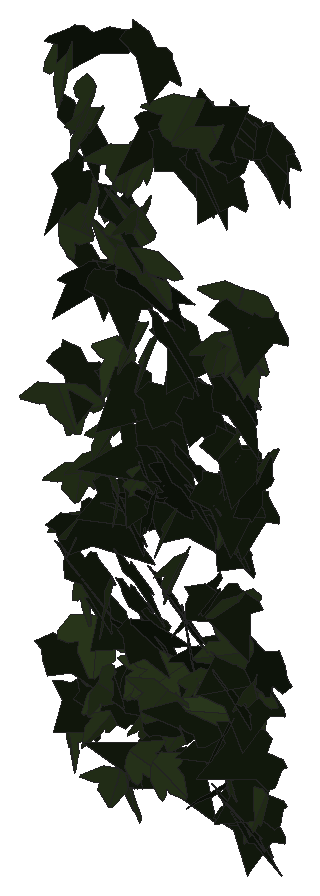
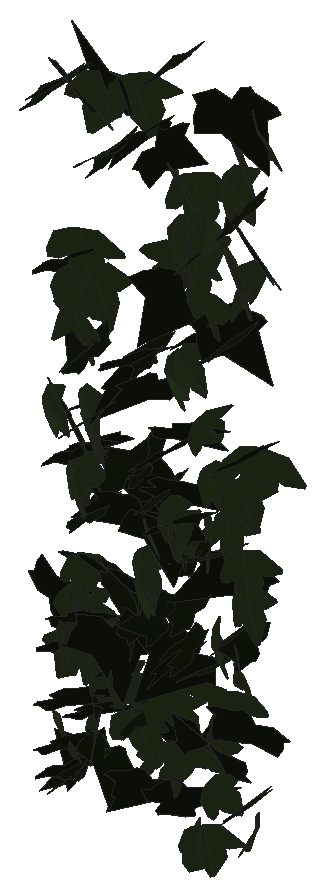
# SketchUp Ruby script. Lengths in inches.
U = 1.inch
M = Sketchup.active_model
def pt(a) = Geom::Point3d.new(a.map { |v| v * U })
def face(e, loops, mat)
  f = e.add_face(loops[0].map { |a| pt(a) })
  loops[1..].each { |l| e.add_face(l.map { |a| pt(a) }).erase! }
  f.material = f.back_material = mat if mat
  f
end
# faces: each face lists its corners as indices into pts; further lists are holes
def faces(e, pts, list, mat = nil) = list.each { |f| face(e, (f[0].is_a?(Array) ? f : [f]).map { |l| l.map { |i| pts[i] } }, mat) }
# xy, xz, yz: faces in a plane at the given z, y or x. An outline is a flat list of corners, or four numbers for a rectangle; further outlines are holes
def ring(l) = l.size == 4 ? [[l[0], l[1]], [l[2], l[1]], [l[2], l[3]], [l[0], l[3]]] : l.each_slice(2).to_a
def flat(e, list, mat, &to3) = list.each { |f| face(e, (f[0].is_a?(Array) ? f : [f]).map { |l| ring(l).map { |u, v| to3.(u, v) } }, mat) }
def xy(e, z, list, mat = nil) = flat(e, list, mat) { |x, y| [x, y, z] }
def xz(e, y, list, mat = nil) = flat(e, list, mat) { |x, z| [x, y, z] }
def yz(e, x, list, mat = nil) = flat(e, list, mat) { |y, z| [x, y, z] }
def lines(e, pts, list) = list.each { |a, b| e.add_line(pt(pts[a]), pt(pts[b])) }
# prism: a flat outline (further loops are holes) pulled along v
def prism(e, loops, v, mat = nil)
  f = face(e, loops, mat); d = Geom::Vector3d.new(v.map { |x| x * U })
  f.pushpull(f.normal.samedirection?(d) ? d.length : -d.length)
end
def box(e, o, s, mat = nil) = prism(e, [[o, [o[0] + s[0], o[1], o[2]], [o[0] + s[0], o[1] + s[1], o[2]], [o[0], o[1] + s[1], o[2]]]], [0, 0, s[2]], mat)
def at(x, y, z, deg = 0) = Geom::Transformation.translation(pt([x, y, z])) * Geom::Transformation.rotation(ORIGIN, Z_AXIS, deg.degrees)
def axes(o, x, y, z) = Geom::Transformation.new([*x, 0, *y, 0, *z, 0, *pt(o).to_a, 1])
def part(name) = M.definitions.add(name)
# library, detail: a bought-in or finely detailed component or shape, given as its bounding box
def library(name, o, s) = part(name).tap { |d| box(d.entities, o, s) }
def detail(e, o, s) = box(e.add_group.entities, o, s)
def put(e, d, t, mat = nil) = e.add_instance(d, t).tap { |i| i.material = mat if mat }
def group(e, t, mat = nil) = e.add_group.tap { |g| g.transformation = t; g.material = mat if mat }.entities
root = M.entities
M.materials.add("1026 AP 7946 SUNNY SIDE UP").color = [254, 231, 186]
M.materials.add("efeu1").color = [18, 25, 13]
M.materials.add("efeu2").color = [43, 57, 29]
c1 = part("ivyleaf_10")
p = [[0,0.5,-0.03],[-0.0625,2.02,-0.43],[-0.19,2.01,-0.46],[-0.54,1.05,-0.29],[-0.52,0.625,-0.18],[-0.83,0.76,-0.28],
  [-1.16,0.64,-0.33],[-1.15,0.33,-0.24],[-0.77,-0.39,0.02],[-0.3,-0.51,0.16],[0.04,-0.48,0.23],[-0.02,2.01,-0.4375],
  [-0.06,2.01,-0.43],[0.04,-0.49,0.23],[0.67,-0.49,0.14],[1.38,0.36,-0.2],[1.375,0.51,-0.24],[0.81,0.65,-0.19],
  [0.62,0.59,-0.15],[0.6,1.09,-0.28],[0.5,1.23,-0.31]]
faces(c1.entities,p,[[0,1,2,3,4,5,6,7,8,9,10],[11,12,0,13,14,15,16,17,18,19,20]],"efeu2")
c2 = part("ivyleaf_9")
p = [[1.54,2.16,1.25],[1.36,2.04,1.19],[-0.21,0.99,0.68],[-0.71,1.11,0.82],[-0.85,0.86,0.67],[-0.8,0.17,0.21],
  [-0.9,-0.01,0.1],[-0.67,-0.16,-0.02],[-0.08,-0.08,-0.05],[-0.03,-0.6,-0.4],[0.65,-0.88,-0.66],[0.83,-0.6,-0.49],
  [1.29,-0.42,-0.43],[1.8125,-0.07,-0.26],[1.21,0.44,0.15]]
faces(c2.entities,p,[[0,1,2,3,4,5,6,7,8,9,10,11,12,13,14]],"efeu1")
put(root,c1,axes([114.49,211.98,276.21],[-0.46755,0.04693,-0.12502],[0.17989,-0.05127,-0.30883],[-0.09827,-0.31714,0.02948]),"1026 AP 7946 SUNNY SIDE UP")
put(root,c1,axes([113.89,211.85,269.51],[0.00016,-0.20597,-0.21313],[0.10425,0.20032,-0.20542],[0.4457,-0.04678,0.04812]),"1026 AP 7946 SUNNY SIDE UP")
put(root,c1,axes([115.85,212.03,275.45],[-0.07822,-0.31944,0.02119],[0.00362,-0.02301,-0.33313],[0.50351,-0.04946,0.00569]),"1026 AP 7946 SUNNY SIDE UP")
put(root,c2,axes([115.95,212.16,268.2],[0.06977,-0.19538,0.20513],[0.16188,-0.1771,-0.20257],[0.40903,0.10342,0.04518]),"1026 AP 7946 SUNNY SIDE UP")
put(root,c1,axes([114.95,211.84,268.58],[-0.00441,0.23066,0.16475],[-0.00701,0.15856,-0.2367],[-0.44011,-0.00484,0.00212]),"1026 AP 7946 SUNNY SIDE UP")
put(root,c1,axes([113.74,212.17,270.73],[0.17168,-0.16437,0.23033],[0.20283,-0.1838,-0.20433],[0.38768,0.16896,0.0049]),"1026 AP 7946 SUNNY SIDE UP")
put(root,c1,axes([116.42,212.08,268.5],[0.29242,-0.22063,0.0544],[0.03417,-0.05227,-0.29707],[0.35554,0.18648,-0.0162]),"1026 AP 7946 SUNNY SIDE UP")
put(root,c1,axes([114.85,212.02,269.61],[-0.38768,-0.02334,0.12794],[-0.18581,-0.05466,-0.25232],[0.07095,-0.27066,0.03826]),"1026 AP 7946 SUNNY SIDE UP")
put(root,c1,axes([114.54,211.85,268.63],[0.06931,0.17777,0.19827],[-0.0026,0.19434,-0.18437],[-0.41079,0.02876,0.03462]),"1026 AP 7946 SUNNY SIDE UP")
put(root,c2,axes([115.3,211.91,270.875],[0.19725,-0.09015,-0.26132],[-0.36298,0.10687,-0.15643],[0.21631,0.26154,-0.02419]),"1026 AP 7946 SUNNY SIDE UP")
put(root,c2,axes([115.85,212.2,270],[0.04597,-0.18928,0.19439],[0.10568,-0.17961,-0.19628],[0.40798,0.06785,0.02894]),"1026 AP 7946 SUNNY SIDE UP")
put(root,c1,axes([113.11,212,273.67],[-0.42995,-0.14829,-0.06151],[0.10163,0.00382,-0.31922],[0.22936,-0.27967,0.02616]),"1026 AP 7946 SUNNY SIDE UP")
put(root,c2,axes([115.88,212.16,273.05],[-0.12212,-0.27707,-0.02042],[0.01419,0.01643,-0.29631],[0.43638,-0.07807,0.00392]),"1026 AP 7946 SUNNY SIDE UP")
put(root,c2,axes([113.99,212.26,270.3],[-0.22655,-0.15842,0.19485],[-0.02833,-0.21261,-0.19791],[0.38799,-0.10803,0.09932]),"1026 AP 7946 SUNNY SIDE UP")
put(root,c2,axes([114.92,212.12,273.1],[0.24743,-0.23517,0.04497],[0.02039,-0.04538,-0.2914],[0.37593,0.15724,-0.0138]),"1026 AP 7946 SUNNY SIDE UP")
put(root,c1,axes([113.35,212.09,271.72],[0.04268,-0.27673,0.03072],[0.00247,-0.03138,-0.28663],[0.43791,0.02715,-0.00138]),"1026 AP 7946 SUNNY SIDE UP")
put(root,c1,axes([113.49,212.07,278.35],[0.26298,-0.28923,-0.02446],[-0.02518,0.01627,-0.34405],[0.45542,0.16791,-0.0049]),"1026 AP 7946 SUNNY SIDE UP")
put(root,c1,axes([112.97,212.1875,278.73],[0.31753,-0.17989,0.18977],[0.19823,-0.13653,-0.27898],[0.35433,0.23759,-0.01398]),"1026 AP 7946 SUNNY SIDE UP")
put(root,c2,axes([113.3,212.15,277.02],[-0.39035,0.08105,-0.18814],[0.25758,-0.08546,-0.26831],[-0.18102,-0.29639,0.02391]),"1026 AP 7946 SUNNY SIDE UP")
put(root,c2,axes([115.99,211.85,269.45],[-0.12678,0.04384,-0.28372],[-0.32819,0.18103,0.09362],[0.2914,0.22297,-0.01801]),"1026 AP 7946 SUNNY SIDE UP")
put(root,c2,axes([115.53,212.22,269.4],[-0.24623,-0.01333,0.22768],[-0.29463,-0.13639,-0.146],[0.18569,-0.23409,0.07026]),"1026 AP 7946 SUNNY SIDE UP")
put(root,c2,axes([115.97,212.26,273.65],[-0.12615,-0.26399,0.08757],[0.01946,-0.09334,-0.28219],[0.43638,-0.07215,0.0379]),"1026 AP 7946 SUNNY SIDE UP")
put(root,c2,axes([113.375,212.18,271.08],[0.11517,-0.29673,0.00737],[-0.00621,-0.01008,-0.31486],[0.46674,0.07308,-0.00601]),"1026 AP 7946 SUNNY SIDE UP")
put(root,c2,axes([113.64,212.13,275.66],[-0.03296,0.21047,-0.24576],[0.02622,-0.23922,-0.21924],[-0.50095,-0.02637,0.00469]),"1026 AP 7946 SUNNY SIDE UP")
put(root,c2,axes([115.52,212.13,278.375],[-0.12133,0.15289,0.29056],[0.18785,-0.25457,0.17488],[0.46688,0.14216,0.00514]),"1026 AP 7946 SUNNY SIDE UP")
put(root,c2,axes([116.31,212.31,269.12],[-0.31889,-0.14425,0.1828],[-0.18201,-0.14103,-0.25406],[0.31126,-0.23025,0.03871]),"1026 AP 7946 SUNNY SIDE UP")
put(root,c2,axes([114.45,212.3125,279.27],[-0.05763,-0.26594,0.15487],[0.00393,-0.15318,-0.27666],[0.48152,-0.03058,0.02079]),"1026 AP 7946 SUNNY SIDE UP")
put(root,c2,axes([114.01,212.28,272.02],[0.07618,-0.18441,0.21341],[0.06247,-0.20458,-0.1974],[0.43285,0.06198,-0.00907]),"1026 AP 7946 SUNNY SIDE UP")
put(root,c1,axes([115.68,212.07,278.49],[-0.40505,-0.19865,-0.0706],[0.10673,0.02207,-0.33411],[0.3121,-0.26535,0.02263]),"1026 AP 7946 SUNNY SIDE UP")
put(root,c2,axes([114.96,212.25,270.76],[0.30141,-0.09309,-0.20331],[0.29183,-0.06726,0.21858],[-0.17901,-0.26638,0.01401]),"1026 AP 7946 SUNNY SIDE UP")
put(root,c2,axes([116.08,212.11,268.14],[0.28891,-0.18786,-0.04595],[-0.05544,0.02639,-0.27047],[0.29811,0.18697,-0.00577]),"1026 AP 7946 SUNNY SIDE UP")
put(root,c2,axes([113.51,211.96,271.91],[-0.01021,-0.06465,-0.32276],[0.12518,0.3028,-0.06438],[0.48661,-0.07926,0.00979]),"1026 AP 7946 SUNNY SIDE UP")
put(root,c1,axes([115.12,212.18,278.69],[-0.29611,-0.25142,0.09091],[-0.0419,-0.09149,-0.32244],[0.41763,-0.18745,0.0321]),"1026 AP 7946 SUNNY SIDE UP")
put(root,c1,axes([113.31,211.89,276.34],[-0.01347,0.18595,0.27429],[-0.11269,0.25763,-0.18698],[-0.49667,-0.0635,0.03499]),"1026 AP 7946 SUNNY SIDE UP")
put(root,c1,axes([114,212.03,272.41],[0.18204,-0.21785,-0.14607],[-0.00546,0.15261,-0.24574],[0.40762,0.09934,0.06194]),"1026 AP 7946 SUNNY SIDE UP")
put(root,c1,axes([114.22,212.25,274.88],[0.05092,-0.26007,0.14748],[0.04114,-0.14244,-0.27072],[0.46611,0.04098,0.00778]),"1026 AP 7946 SUNNY SIDE UP")
put(root,c1,axes([115.56,212.25,269.5],[-0.08745,0.07249,0.26375],[-0.25602,-0.21566,0.02525],[0.33013,-0.14805,0.08945]),"1026 AP 7946 SUNNY SIDE UP")
put(root,c2,axes([113.88,212.28,275.52],[-0.02287,-0.30449,0.02906],[-0.00042,-0.02996,-0.31422],[0.48109,-0.0145,0.0011]),"1026 AP 7946 SUNNY SIDE UP")
put(root,c1,axes([116.18,212.25,275.45],[-0.10318,-0.24931,0.14987],[-0.03804,-0.14537,-0.26616],[0.45341,-0.06893,0.01178]),"1026 AP 7946 SUNNY SIDE UP")
put(root,c2,axes([116.2,212.27,268.13],[-0.13827,-0.25698,0.015],[0.00443,-0.01789,-0.27978],[0.40484,-0.08758,0.00819]),"1026 AP 7946 SUNNY SIDE UP")
put(root,c2,axes([114.68,212.18,272.68],[0.14344,-0.05207,0.27289],[0.3296,-0.16303,-0.10822],[0.26823,0.22818,-0.01296]),"1026 AP 7946 SUNNY SIDE UP")
put(root,c2,axes([113.07,212.22,271.02],[0.25099,-0.21041,0.08354],[0.05945,-0.07446,-0.27212],[0.35024,0.16342,-0.01368]),"1026 AP 7946 SUNNY SIDE UP")
put(root,c2,axes([115.86,212.34,269.1],[-0.28199,-0.09829,0.18486],[-0.18036,-0.15014,-0.20307],[0.26732,-0.20499,0.05799]),"1026 AP 7946 SUNNY SIDE UP")
put(root,c2,axes([116.32,212.35,268.45],[-0.25498,-0.15213,0.15768],[-0.12726,-0.13574,-0.22686],[0.31559,-0.17765,0.03591]),"1026 AP 7946 SUNNY SIDE UP")
put(root,c1,axes([115.88,212.07,268.78],[-0.2182,0.22179,0.07135],[-0.098,0.04068,-0.26748],[-0.35135,-0.14908,0.03029]),"1026 AP 7946 SUNNY SIDE UP")
put(root,c2,axes([116.17,212.32,275.8],[-0.16645,-0.27761,0.02002],[0.00377,-0.02339,-0.30602],[0.43775,-0.10536,0.01025]),"1026 AP 7946 SUNNY SIDE UP")
put(root,c2,axes([113.15,212.16,269.76],[-0.07612,-0.14172,-0.26228],[0.3244,0.1645,-0.13421],[0.32198,-0.19924,0.07321]),"1026 AP 7946 SUNNY SIDE UP")
put(root,c1,axes([116.09,212.21,270.64],[-0.22466,-0.04339,0.26123],[-0.35516,-0.11827,-0.1525],[0.19443,-0.26617,0.02327]),"1026 AP 7946 SUNNY SIDE UP")
put(root,c2,axes([114.0625,212.28,271.1875],[0.17915,-0.22704,0.11541],[0.06852,-0.10486,-0.2622],[0.39306,0.12176,-0.00689]),"1026 AP 7946 SUNNY SIDE UP")
put(root,c2,axes([113.875,212.29,276.73],[0.10515,-0.29695,0.03704],[-0.00037,-0.03862,-0.31367],[0.47066,0.06631,-0.00852]),"1026 AP 7946 SUNNY SIDE UP")
put(root,c1,axes([115.85,212.32,272.73],[-0.02744,-0.21768,0.19612],[0.0818,-0.19119,-0.22],[0.44859,0.02155,0.05212]),"1026 AP 7946 SUNNY SIDE UP")
put(root,c2,axes([114.39,212.14,269.125],[-0.1717,0.14195,0.27367],[0.29961,-0.18517,0.1821],[0.36534,0.21857,-0.02073]),"1026 AP 7946 SUNNY SIDE UP")
put(root,c2,axes([115.36,212.05,274.29],[0.16756,-0.17896,-0.25689],[-0.19975,0.21339,-0.21332],[0.43791,0.16581,0.00099]),"1026 AP 7946 SUNNY SIDE UP")
put(root,c2,axes([114.95,212.21,278.08],[0.09111,-0.30461,-0.11204],[-0.02654,0.10573,-0.3188],[0.50697,0.06028,0.00345]),"1026 AP 7946 SUNNY SIDE UP")
put(root,c1,axes([114.76,212.28,272.22],[0.16562,-0.23316,0.1238],[0.05849,-0.11636,-0.26393],[0.40925,0.11099,-0.01238]),"1026 AP 7946 SUNNY SIDE UP")
put(root,c1,axes([114.32,212.1,276.54],[-0.29457,0.04892,-0.26597],[-0.36974,0.11106,0.19789],[0.18537,0.29926,-0.02793]),"1026 AP 7946 SUNNY SIDE UP")
put(root,c2,axes([114.85,212.08,274.3],[0.09193,-0.18633,-0.23931],[0.02197,0.23714,-0.19183],[0.46644,0.02556,0.0562]),"1026 AP 7946 SUNNY SIDE UP")
put(root,c1,axes([114.29,212.17,276.77],[-0.00488,-0.31759,-0.0343],[0.00653,0.03145,-0.32699],[0.50179,-0.0035,0.00392]),"1026 AP 7946 SUNNY SIDE UP")
put(root,c1,axes([113.38,212.29,277.87],[0.01818,-0.29185,0.13558],[0.02889,-0.13253,-0.30143],[0.50366,0.01814,0.0124]),"1026 AP 7946 SUNNY SIDE UP")
put(root,c2,axes([116.53,211.97,273.37],[-0.23333,0.04716,-0.30152],[-0.41909,0.12277,0.16017],[0.20506,0.30458,-0.01576]),"1026 AP 7946 SUNNY SIDE UP")
put(root,c2,axes([114.92,212.38,269.25],[-0.05002,-0.17703,0.21674],[0.06438,-0.21347,-0.17907],[0.42876,0.0114,0.05217]),"1026 AP 7946 SUNNY SIDE UP")
put(root,c2,axes([115.62,212.25,271.3125],[-0.1614,-0.17412,-0.20265],[0.31254,0.08516,-0.18493],[0.2683,-0.20394,0.09352]),"1026 AP 7946 SUNNY SIDE UP")
put(root,c2,axes([116.62,212.06,270.43],[0.0342,-0.03002,0.30632],[-0.23398,0.25766,0.0395],[-0.40784,-0.15034,0.00303]),"1026 AP 7946 SUNNY SIDE UP")
put(root,c1,axes([113.77,212.25,273.3],[-0.02669,-0.27337,0.07978],[-0.0086,-0.07881,-0.28263],[0.44736,-0.01782,-0.00067]),"1026 AP 7946 SUNNY SIDE UP")
put(root,c2,axes([116.01,212.33,272.97],[-0.12563,-0.28007,0.01122],[0.00575,-0.01402,-0.30002],[0.44078,-0.07964,0.00711]),"1026 AP 7946 SUNNY SIDE UP")
put(root,c1,axes([114.35,212.34,274.67],[0.18237,-0.206,0.19581],[0.12986,-0.17278,-0.24434],[0.42247,0.14203,-0.00942]),"1026 AP 7946 SUNNY SIDE UP")
put(root,c2,axes([115.83,212.26,274.54],[0.11102,-0.27987,-0.03842],[-0.03125,0.03178,-0.29694],[0.44253,0.07246,-0.01133]),"1026 AP 7946 SUNNY SIDE UP")
put(root,c2,axes([114.41,212.08,275.81],[0.46875,0.06205,-0.05582],[-0.07525,-0.03675,-0.31278],[-0.10587,0.30082,-0.02484]),"1026 AP 7946 SUNNY SIDE UP")
put(root,c1,axes([114.92,212.23,271.625],[0.01355,-0.29129,0.02442],[-0.00187,-0.02541,-0.30036],[0.45975,0.00848,-0.00194]),"1026 AP 7946 SUNNY SIDE UP")
put(root,c2,axes([116.05,212.36,270.45],[-0.34372,-0.15109,0.09497],[-0.09282,-0.07731,-0.27264],[0.26312,-0.22464,0.02788]),"1026 AP 7946 SUNNY SIDE UP")
put(root,c2,axes([116.06,212.31,269.99],[-0.23945,-0.22061,-0.06469],[0.09933,0.03058,-0.27378],[0.34616,-0.16138,0.03381]),"1026 AP 7946 SUNNY SIDE UP")
put(root,c1,axes([113.51,212.22,270.08],[0.47409,0.09148,0.01457],[0.03107,-0.01834,-0.32381],[-0.14206,0.30126,-0.02221]),"1026 AP 7946 SUNNY SIDE UP")
put(root,c2,axes([115.68,212.02,268.43],[0.04162,0.26217,0.06305],[0.00271,0.05984,-0.27107],[-0.42279,0.02619,0.00447]),"1026 AP 7946 SUNNY SIDE UP")
put(root,c1,axes([116.02,212.21,276.08],[-0.41937,-0.11855,0.05922],[-0.06287,-0.05242,-0.29928],[0.19788,-0.26789,0.03043]),"1026 AP 7946 SUNNY SIDE UP")
put(root,c1,axes([114.35,212.26,277.66],[0.33162,-0.27042,0.01062],[-0.01148,-0.0207,-0.3529],[0.42546,0.21021,-0.0178]),"1026 AP 7946 SUNNY SIDE UP")
put(root,c1,axes([114.06,212.22,277.59],[-0.28765,-0.2639,0.01735],[0.01065,-0.02697,-0.33026],[0.41582,-0.18187,0.02047]),"1026 AP 7946 SUNNY SIDE UP")
put(root,c1,axes([114.8,212.25,269.87],[0.40913,-0.00443,-0.15975],[-0.24331,-0.02812,-0.26687],[-0.01668,0.30158,-0.02546]),"1026 AP 7946 SUNNY SIDE UP")
put(root,c2,axes([114.26,212.09,270.41],[0.48433,0.08456,-0.00381],[0.00611,-0.02987,-0.3278],[-0.13298,0.3066,-0.02894]),"1026 AP 7946 SUNNY SIDE UP")
put(root,c2,axes([115.72,212.4375,272.09],[-0.13274,-0.1676,0.22981],[0.011,-0.2352,-0.17993],[0.43979,-0.04471,0.07386]),"1026 AP 7946 SUNNY SIDE UP")
put(root,c1,axes([115.07,212.23,269.18],[-0.33823,-0.121,0.10108],[-0.12385,-0.0612,-0.25422],[0.21213,-0.22866,0.01274]),"1026 AP 7946 SUNNY SIDE UP")
put(root,c2,axes([113.98,212.42,272.08],[-0.32255,-0.09937,0.16937],[-0.08355,-0.20247,-0.19488],[0.29107,-0.16823,0.13175]),"1026 AP 7946 SUNNY SIDE UP")
put(root,c2,axes([115.51,212.4375,277.66],[-0.16719,-0.24119,0.15279],[-0.02479,-0.15457,-0.26904],[0.44566,-0.09908,0.04235]),"1026 AP 7946 SUNNY SIDE UP")
put(root,c2,axes([114.53,212.43,278.1],[-0.00969,0.00304,-0.334],[0.19043,-0.3008,-0.00703],[-0.47294,-0.12118,0.00401]),"1026 AP 7946 SUNNY SIDE UP")
put(root,c1,axes([113.17,212.25,271.66],[-0.06525,-0.28072,0.02025],[0.0005,-0.02152,-0.29244],[0.44266,-0.04135,0.00332]),"1026 AP 7946 SUNNY SIDE UP")
put(root,c2,axes([114.26,212.4,273.94],[-0.36925,-0.15721,0.06137],[-0.05208,-0.05861,-0.28987],[0.25968,-0.2353,0.02913]),"1026 AP 7946 SUNNY SIDE UP")
put(root,c2,axes([114.33,212.18,270.41],[0.13926,-0.21898,-0.19317],[-0.09873,0.17546,-0.24224],[0.44113,0.1084,0.00676]),"1026 AP 7946 SUNNY SIDE UP")
put(root,c1,axes([115.82,212.28,273.42],[0.17046,-0.26571,0.0245],[0.00222,-0.02673,-0.29566],[0.41969,0.10806,-0.00839]),"1026 AP 7946 SUNNY SIDE UP")
put(root,c1,axes([113.49,212.22,272.73],[-0.11207,-0.27856,-0.04915],[0.03912,0.04119,-0.29564],[0.44225,-0.07423,0.01369]),"1026 AP 7946 SUNNY SIDE UP")
put(root,c1,axes([116.25,212.16,270.2],[-0.02326,-0.24599,-0.14891],[0.02981,0.14217,-0.25287],[0.44652,-0.0223,0.00912]),"1026 AP 7946 SUNNY SIDE UP")
put(root,c2,axes([114.46,212.37,268.23],[-0.11768,0.0014,0.27317],[-0.3952,-0.08818,-0.07312],[0.13287,-0.26103,0.02446]),"1026 AP 7946 SUNNY SIDE UP")
put(root,c1,axes([115.22,212.375,269.85],[-0.01196,-0.2398,0.14704],[0.02597,-0.14428,-0.2473],[0.43913,0.00201,0.01863]),"1026 AP 7946 SUNNY SIDE UP")
put(root,c1,axes([114.45,212.36,269.7],[-0.27173,-0.11601,0.1695],[-0.12579,-0.16029,-0.20312],[0.29141,-0.17737,0.07037]),"1026 AP 7946 SUNNY SIDE UP")
put(root,c1,axes([116.05,212.26,272.58],[0.04387,-0.2895,-0.02645],[-0.0055,0.02381,-0.29948],[0.45674,0.02809,-0.00107]),"1026 AP 7946 SUNNY SIDE UP")
put(root,c2,axes([115.43,212.33,271.28],[-0.29415,0.14107,-0.15837],[0.16168,-0.11855,-0.24042],[-0.28654,-0.21171,0.02692]),"1026 AP 7946 SUNNY SIDE UP")
put(root,c1,axes([116.07,212.25,274.94],[0.3506,-0.17854,-0.08279],[-0.08158,0.06198,-0.29348],[0.29618,0.22841,0.01717]),"1026 AP 7946 SUNNY SIDE UP")
put(root,c2,axes([115.75,212.48,273.56],[-0.09297,-0.25627,0.14066],[-0.0266,-0.13754,-0.27143],[0.4569,-0.06015,0.01282]),"1026 AP 7946 SUNNY SIDE UP")
put(root,c1,axes([113.17,212.38,270.64],[0.21838,-0.13518,0.20239],[0.25222,-0.11647,-0.19929],[0.27882,0.21124,0.02176]),"1026 AP 7946 SUNNY SIDE UP")
put(root,c1,axes([113.4,212.27,276.66],[0.2788,-0.27954,-0.07121],[-0.06076,0.05547,-0.34069],[0.4481,0.18145,-0.00189]),"1026 AP 7946 SUNNY SIDE UP")
put(root,c1,axes([113.58,212.42,268.72],[-0.05823,-0.18897,0.19337],[0.00171,-0.19069,-0.19755],[0.42,-0.02542,0.02761]),"1026 AP 7946 SUNNY SIDE UP")
put(root,c2,axes([114.49,212.4,272.96],[-0.40496,-0.03107,0.1612],[-0.23685,-0.05152,-0.26594],[0.08345,-0.29701,0.02746]),"1026 AP 7946 SUNNY SIDE UP")
put(root,c2,axes([113.15,212.46,273.9],[-0.10284,-0.27208,0.0823],[-0.00553,-0.08279,-0.28833],[0.44654,-0.06369,0.01539]),"1026 AP 7946 SUNNY SIDE UP")
put(root,c1,axes([113.83,212.3,267.91],[-0.28729,-0.18059,0.03552],[-0.02196,-0.03628,-0.26436],[0.28856,-0.18255,0.01525]),"1026 AP 7946 SUNNY SIDE UP")
put(root,c2,axes([115.03,212.46,273.01],[0.063,-0.22576,0.19194],[0.12793,-0.17337,-0.23386],[0.44346,0.08208,0.0402]),"1026 AP 7946 SUNNY SIDE UP")
put(root,c1,axes([113.71,212.37,269.25],[0.25873,0.13618,-0.1651],[-0.1825,-0.11206,-0.22046],[-0.27688,0.20112,-0.00897]),"1026 AP 7946 SUNNY SIDE UP")
put(root,c1,axes([114.3125,212.4375,272.66],[-0.02573,-0.21482,0.18919],[0.02007,-0.18554,-0.22204],[0.44519,-0.00405,0.02094]),"1026 AP 7946 SUNNY SIDE UP")
put(root,c2,axes([113.11,212.51,268.6],[-0.16046,-0.14633,0.21381],[-0.06959,-0.21088,-0.17612],[0.39428,-0.09677,0.05593]),"1026 AP 7946 SUNNY SIDE UP")
put(root,c1,axes([112.98,212.34,268.3125],[-0.06259,0.23569,-0.11815],[0.03526,-0.11387,-0.24689],[-0.41157,-0.0456,-0.00318]),"1026 AP 7946 SUNNY SIDE UP")
put(root,c2,axes([115.875,212.3,268.26],[0.16988,-0.21924,-0.08883],[-0.04311,0.08114,-0.25108],[0.3672,0.11095,0.01162]),"1026 AP 7946 SUNNY SIDE UP")
put(root,c2,axes([114.59,212.42,274.98],[0.17144,-0.26375,0.07378],[0.02641,-0.0721,-0.29419],[0.42954,0.1097,-0.01136]),"1026 AP 7946 SUNNY SIDE UP")
put(root,c2,axes([115.26,212.46,277.76],[0.08598,-0.28808,0.07874],[0.008,-0.07845,-0.30238],[0.46925,0.05412,-0.00927]),"1026 AP 7946 SUNNY SIDE UP")
put(root,c1,axes([114.17,212.45,272.47],[0.02334,-0.23864,0.17772],[0.07372,-0.16997,-0.24546],[0.45838,0.03949,0.03043]),"1026 AP 7946 SUNNY SIDE UP")
put(root,c2,axes([113.38,212.3,279.13],[0.0893,0.23861,-0.21236],[-0.06728,-0.20307,-0.25383],[-0.49263,0.07098,-0.00383]),"1026 AP 7946 SUNNY SIDE UP")
put(root,c1,axes([116.34,212.43,273.59],[0.12569,-0.24299,0.13366],[0.05628,-0.12623,-0.26422],[0.43049,0.08745,-0.00448]),"1026 AP 7946 SUNNY SIDE UP")
put(root,c1,axes([115.8125,212.34,273.78],[0.09996,-0.2821,-0.00091],[-0.0042,-0.00134,-0.2979],[0.44355,0.06356,-0.00261]),"1026 AP 7946 SUNNY SIDE UP")
put(root,c2,axes([113.34,212.51,275.53],[-0.0203,-0.27343,0.1281],[0.03367,-0.12653,-0.28157],[0.47212,-0.00273,0.02559]),"1026 AP 7946 SUNNY SIDE UP")
put(root,c2,axes([116.21,212.1,278.34],[-0.38447,0.0994,-0.21042],[-0.2739,0.11184,0.2708],[0.2305,0.29871,-0.02919]),"1026 AP 7946 SUNNY SIDE UP")
put(root,c2,axes([114.46,212.09,272.13],[0.04028,0.0144,0.32673],[0.0323,0.31736,-0.0147],[-0.49803,0.02175,0.02547]),"1026 AP 7946 SUNNY SIDE UP")
put(root,c2,axes([115.65,212.5,274.6],[0.06367,-0.22264,0.19559],[0.11335,-0.17947,-0.23216],[0.44723,0.07718,0.031]),"1026 AP 7946 SUNNY SIDE UP")
put(root,c2,axes([114.57,212.24,272.42],[0.26196,0.16906,-0.16081],[-0.19811,-0.09565,-0.24431],[-0.30398,0.20803,0.02064]),"1026 AP 7946 SUNNY SIDE UP")
put(root,c1,axes([115.97,212.2,275.28],[-0.16087,-0.2474,-0.2029],[0.17678,0.16346,-0.27268],[0.46327,-0.14828,0.0336]),"1026 AP 7946 SUNNY SIDE UP")
put(root,c2,axes([114.23,212.52,272.58],[-0.19814,-0.24468,0.08145],[-0.02626,-0.08161,-0.28313],[0.40414,-0.12526,0.02153]),"1026 AP 7946 SUNNY SIDE UP")
put(root,c2,axes([116.1875,212.4,278.54],[0.07765,-0.29902,-0.05659],[0.01023,0.05497,-0.31151],[0.47746,0.04745,0.01588]),"1026 AP 7946 SUNNY SIDE UP")
put(root,c1,axes([113.7,212.53,274.23],[-0.11543,-0.18657,0.24237],[0.12819,-0.24647,-0.17582],[0.45575,0.02207,0.11084]),"1026 AP 7946 SUNNY SIDE UP")
put(root,c2,axes([114.92,212.33,272.46],[-0.01039,-0.16966,-0.28622],[0.36207,0.19281,-0.12625],[0.36001,-0.19881,0.11872]),"1026 AP 7946 SUNNY SIDE UP")
put(root,c2,axes([113.78,212.22,268.98],[-0.3352,0.13823,0.19471],[0.27564,-0.07365,0.25983],[0.2426,0.27467,-0.02619]),"1026 AP 7946 SUNNY SIDE UP")
put(root,c1,axes([115.73,212.28,270.17],[-0.17831,-0.24117,-0.08157],[0.06767,0.06568,-0.27394],[0.39267,-0.12083,0.01016]),"1026 AP 7946 SUNNY SIDE UP")
put(root,c2,axes([115.46,212.24,270.41],[0.15983,0.26544,-0.11638],[-0.05194,-0.10989,-0.29335],[-0.45156,0.10659,-0.00745]),"1026 AP 7946 SUNNY SIDE UP")
put(root,c1,axes([114.12,212.29,267.53],[-0.27307,0.20972,-0.0371],[-0.02027,0.03757,0.28037],[0.33431,0.17359,-0.0133]),"1026 AP 7946 SUNNY SIDE UP")
put(root,c2,axes([113.98,212.42,270.7],[0.21557,-0.2329,0.05522],[0.02956,-0.05262,-0.27852],[0.37509,0.138,-0.00978]),"1026 AP 7946 SUNNY SIDE UP")
put(root,c1,axes([115.87,212.3125,271.29],[-0.16884,-0.25448,-0.07241],[0.0583,0.05901,-0.28398],[0.41041,-0.11308,0.01055]),"1026 AP 7946 SUNNY SIDE UP")
put(root,c1,axes([113.78,212.13,276.75],[0.10288,-0.07957,0.31111],[-0.21798,0.2696,0.10554],[-0.44079,-0.15189,0.02042]),"1026 AP 7946 SUNNY SIDE UP")
put(root,c2,axes([114.74,212.33,268.43],[-0.10686,-0.14899,-0.23509],[0.18179,0.19626,-0.16694],[0.38683,-0.13339,0.01351]),"1026 AP 7946 SUNNY SIDE UP")
put(root,c2,axes([113.02,212.54,277.62],[0.07063,-0.28146,0.12023],[0.02343,-0.11741,-0.2943],[0.47951,0.04719,-0.00333]),"1026 AP 7946 SUNNY SIDE UP")
put(root,c1,axes([113.15,212.43,273.4],[-0.17357,-0.25238,0.07884],[-0.018,-0.07984,-0.28345],[0.41495,-0.10903,0.02068]),"1026 AP 7946 SUNNY SIDE UP")
put(root,c1,axes([114,212.22,275.87],[-0.1434,0.05672,-0.31138],[-0.34378,0.21023,0.10971],[0.34078,0.23595,-0.02035]),"1026 AP 7946 SUNNY SIDE UP")
put(root,c1,axes([114.75,212.48,271.41],[0.12644,-0.24034,0.12105],[0.05948,-0.11269,-0.26175],[0.41739,0.08886,0.00063]),"1026 AP 7946 SUNNY SIDE UP")
put(root,c2,axes([116.22,212.56,278.43],[0.00578,-0.29741,0.1047],[0.03636,-0.10279,-0.30627],[0.49372,0.01105,0.02133]),"1026 AP 7946 SUNNY SIDE UP")
put(root,c1,axes([114.31,212.35,269.01],[0.00208,-0.26557,-0.05947],[0.03034,0.05617,-0.27255],[0.42576,-0.0027,0.01972]),"1026 AP 7946 SUNNY SIDE UP")
put(root,c2,axes([114.38,212.4,272.99],[0.21007,-0.24321,-0.066],[-0.04212,0.05679,-0.28551],[0.39267,0.13621,0.00468]),"1026 AP 7946 SUNNY SIDE UP")
put(root,c1,axes([116.03,212.375,270.01],[-0.3815,0.09516,-0.06789],[0.06891,-0.06745,-0.26478],[-0.16899,-0.24234,0.0453]),"1026 AP 7946 SUNNY SIDE UP")
put(root,c2,axes([114.44,212.42,273.54],[0.09825,-0.27899,-0.0844],[0.00903,0.08335,-0.29309],[0.45642,0.05841,0.02397]),"1026 AP 7946 SUNNY SIDE UP")
put(root,c2,axes([114.4375,212.4375,271.05],[0.28965,-0.2007,0.05332],[0.02905,-0.05458,-0.27998],[0.32506,0.18371,-0.02249]),"1026 AP 7946 SUNNY SIDE UP")
put(root,c2,axes([114.97,212.58,274.83],[-0.22516,-0.23626,0.10151],[-0.03757,-0.1016,-0.28348],[0.40157,-0.14197,0.03039]),"1026 AP 7946 SUNNY SIDE UP")
put(root,c1,axes([113.1,212.38,272.32],[-0.21227,-0.24741,-0.00732],[0.01837,0.00011,-0.29016],[0.3887,-0.13512,0.00972]),"1026 AP 7946 SUNNY SIDE UP")
